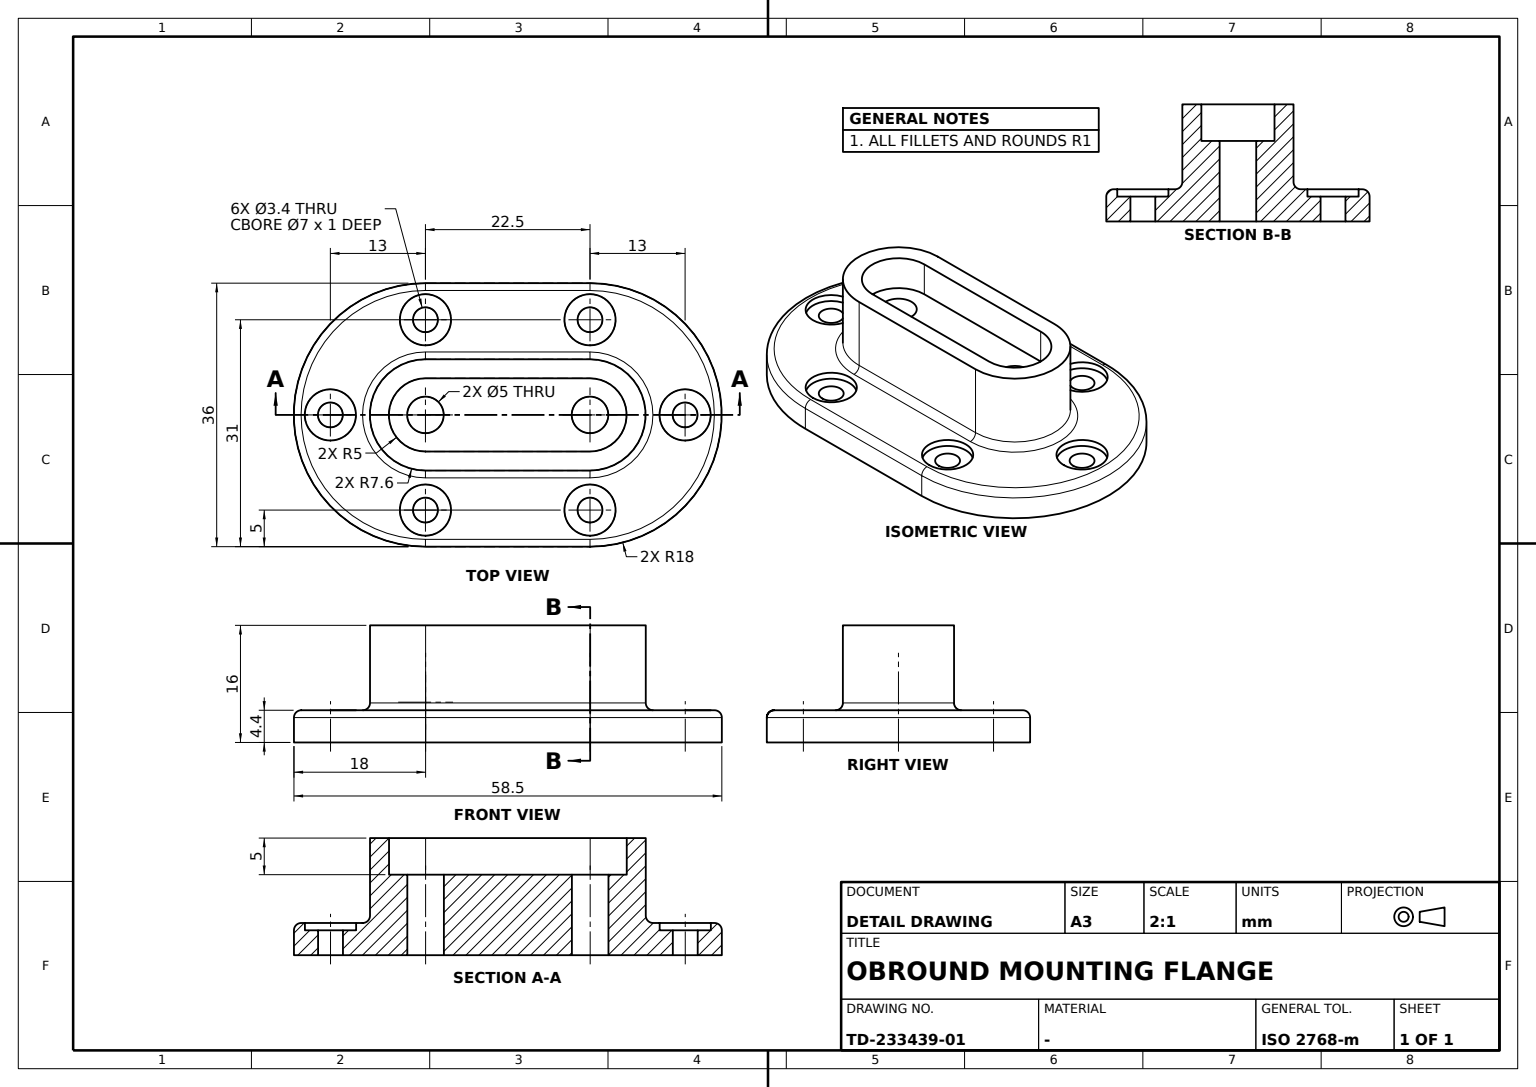
ISO-10303-21;
HEADER;
FILE_DESCRIPTION((''),'2;1');
FILE_NAME('','',(''),(''),'','','');
FILE_SCHEMA(('AUTOMOTIVE_DESIGN'));
ENDSEC;
DATA;
#1=APPLICATION_CONTEXT('');
#2=PRODUCT_CONTEXT('',#1,'mechanical');
#3=PRODUCT('','','',(#2));
#4=PRODUCT_DEFINITION_FORMATION('','',#3);
#5=PRODUCT_DEFINITION_CONTEXT('',#1,'design');
#6=PRODUCT_DEFINITION('','',#4,#5);
#7=PRODUCT_DEFINITION_SHAPE('','',#6);
#8=(LENGTH_UNIT()NAMED_UNIT(*)SI_UNIT(.MILLI.,.METRE.));
#9=(NAMED_UNIT(*)PLANE_ANGLE_UNIT()SI_UNIT($,.RADIAN.));
#10=(NAMED_UNIT(*)SI_UNIT($,.STERADIAN.)SOLID_ANGLE_UNIT());
#11=UNCERTAINTY_MEASURE_WITH_UNIT(LENGTH_MEASURE(0.005),#8,'distance_accuracy_value','');
#12=(GEOMETRIC_REPRESENTATION_CONTEXT(3)GLOBAL_UNCERTAINTY_ASSIGNED_CONTEXT((#11))GLOBAL_UNIT_ASSIGNED_CONTEXT((#8,#9,#10))REPRESENTATION_CONTEXT('',''));
#13=CARTESIAN_POINT('',(-8.6,-11.25,2.2));
#14=VERTEX_POINT('',#13);
#15=CARTESIAN_POINT('',(-7.6,-11.25,3.2));
#16=VERTEX_POINT('',#15);
#17=CARTESIAN_POINT('',(-8.6,-11.25,3.2));
#18=DIRECTION('',(0.,1.,0.));
#19=DIRECTION('',(0.,0.,1.));
#20=AXIS2_PLACEMENT_3D('',#17,#18,#19);
#21=CIRCLE('',#20,1.);
#22=EDGE_CURVE('',#14,#16,#21,.F.);
#23=ORIENTED_EDGE('',*,*,#22,.F.);
#24=CARTESIAN_POINT('',(8.6,-11.25,2.2));
#25=VERTEX_POINT('',#24);
#26=CARTESIAN_POINT('',(0.,-11.25,2.2));
#27=DIRECTION('',(1.,0.,0.));
#28=AXIS2_PLACEMENT_3D('',#26,#19,#27);
#29=CIRCLE('',#28,8.6);
#30=EDGE_CURVE('',#14,#25,#29,.T.);
#31=ORIENTED_EDGE('',*,*,#30,.T.);
#32=CARTESIAN_POINT('',(7.6,-11.25,3.2));
#33=VERTEX_POINT('',#32);
#34=CARTESIAN_POINT('',(8.6,-11.25,3.2));
#35=AXIS2_PLACEMENT_3D('',#34,#18,#19);
#36=CIRCLE('',#35,1.);
#37=EDGE_CURVE('',#25,#33,#36,.T.);
#38=ORIENTED_EDGE('',*,*,#37,.T.);
#39=CARTESIAN_POINT('',(0.,-11.25,3.2));
#40=AXIS2_PLACEMENT_3D('',#39,#19,#27);
#41=CIRCLE('',#40,7.6);
#42=EDGE_CURVE('',#16,#33,#41,.T.);
#43=ORIENTED_EDGE('',*,*,#42,.F.);
#44=EDGE_LOOP('',(#23,#31,#38,#43));
#45=FACE_BOUND('',#44,.T.);
#46=DIRECTION('',(-0.691222874,0.722641639,0.));
#47=AXIS2_PLACEMENT_3D('',#39,#19,#46);
#48=TOROIDAL_SURFACE('',#47,8.6,1.);
#49=ADVANCED_FACE('',(#45),#48,.F.);
#50=CARTESIAN_POINT('',(7.6,11.25,3.2));
#51=VERTEX_POINT('',#50);
#52=CARTESIAN_POINT('',(7.6,11.25,13.8));
#53=VERTEX_POINT('',#52);
#54=CARTESIAN_POINT('',(7.6,11.25,8.));
#55=VECTOR('',#19,1000.);
#56=LINE('',#54,#55);
#57=EDGE_CURVE('',#51,#53,#56,.T.);
#58=ORIENTED_EDGE('',*,*,#57,.T.);
#59=CARTESIAN_POINT('',(7.6,-11.25,13.8));
#60=VERTEX_POINT('',#59);
#61=CARTESIAN_POINT('',(7.6,0.,13.8));
#62=VECTOR('',#18,1000.);
#63=LINE('',#61,#62);
#64=EDGE_CURVE('',#60,#53,#63,.T.);
#65=ORIENTED_EDGE('',*,*,#64,.F.);
#66=CARTESIAN_POINT('',(7.6,-11.25,8.));
#67=LINE('',#66,#55);
#68=EDGE_CURVE('',#33,#60,#67,.T.);
#69=ORIENTED_EDGE('',*,*,#68,.F.);
#70=CARTESIAN_POINT('',(7.6,0.,3.2));
#71=LINE('',#70,#62);
#72=EDGE_CURVE('',#33,#51,#71,.T.);
#73=ORIENTED_EDGE('',*,*,#72,.T.);
#74=EDGE_LOOP('',(#58,#65,#69,#73));
#75=FACE_BOUND('',#74,.T.);
#76=CARTESIAN_POINT('',(7.6,-11.25,2.2));
#77=AXIS2_PLACEMENT_3D('',#76,#27,#18);
#78=PLANE('',#77);
#79=ADVANCED_FACE('',(#75),#78,.T.);
#80=CARTESIAN_POINT('',(2.5,-11.25,-2.2));
#81=VERTEX_POINT('',#80);
#82=CARTESIAN_POINT('',(0.,-11.25,-2.2));
#83=AXIS2_PLACEMENT_3D('',#82,#19,#27);
#84=CIRCLE('',#83,2.5);
#85=EDGE_CURVE('',#81,#81,#84,.T.);
#86=ORIENTED_EDGE('',*,*,#85,.T.);
#87=EDGE_LOOP('',(#86));
#88=FACE_BOUND('',#87,.T.);
#89=CARTESIAN_POINT('',(1.7,24.25,-2.2));
#90=VERTEX_POINT('',#89);
#91=CARTESIAN_POINT('',(0.,24.25,-2.2));
#92=AXIS2_PLACEMENT_3D('',#91,#19,#27);
#93=CIRCLE('',#92,1.7);
#94=EDGE_CURVE('',#90,#90,#93,.T.);
#95=ORIENTED_EDGE('',*,*,#94,.T.);
#96=EDGE_LOOP('',(#95));
#97=FACE_BOUND('',#96,.T.);
#98=CARTESIAN_POINT('',(2.5,11.25,-2.2));
#99=VERTEX_POINT('',#98);
#100=CARTESIAN_POINT('',(0.,11.25,-2.2));
#101=AXIS2_PLACEMENT_3D('',#100,#19,#27);
#102=CIRCLE('',#101,2.5);
#103=EDGE_CURVE('',#99,#99,#102,.T.);
#104=ORIENTED_EDGE('',*,*,#103,.T.);
#105=EDGE_LOOP('',(#104));
#106=FACE_BOUND('',#105,.T.);
#107=CARTESIAN_POINT('',(-11.3,11.25,-2.2));
#108=VERTEX_POINT('',#107);
#109=CARTESIAN_POINT('',(-13.,11.25,-2.2));
#110=AXIS2_PLACEMENT_3D('',#109,#19,#27);
#111=CIRCLE('',#110,1.7);
#112=EDGE_CURVE('',#108,#108,#111,.T.);
#113=ORIENTED_EDGE('',*,*,#112,.T.);
#114=EDGE_LOOP('',(#113));
#115=FACE_BOUND('',#114,.T.);
#116=CARTESIAN_POINT('',(14.7,11.25,-2.2));
#117=VERTEX_POINT('',#116);
#118=CARTESIAN_POINT('',(13.,11.25,-2.2));
#119=AXIS2_PLACEMENT_3D('',#118,#19,#27);
#120=CIRCLE('',#119,1.7);
#121=EDGE_CURVE('',#117,#117,#120,.T.);
#122=ORIENTED_EDGE('',*,*,#121,.T.);
#123=EDGE_LOOP('',(#122));
#124=FACE_BOUND('',#123,.T.);
#125=CARTESIAN_POINT('',(1.7,-24.25,-2.2));
#126=VERTEX_POINT('',#125);
#127=CARTESIAN_POINT('',(0.,-24.25,-2.2));
#128=AXIS2_PLACEMENT_3D('',#127,#19,#27);
#129=CIRCLE('',#128,1.7);
#130=EDGE_CURVE('',#126,#126,#129,.T.);
#131=ORIENTED_EDGE('',*,*,#130,.T.);
#132=EDGE_LOOP('',(#131));
#133=FACE_BOUND('',#132,.T.);
#134=CARTESIAN_POINT('',(14.7,-11.25,-2.2));
#135=VERTEX_POINT('',#134);
#136=CARTESIAN_POINT('',(13.,-11.25,-2.2));
#137=AXIS2_PLACEMENT_3D('',#136,#19,#27);
#138=CIRCLE('',#137,1.7);
#139=EDGE_CURVE('',#135,#135,#138,.T.);
#140=ORIENTED_EDGE('',*,*,#139,.T.);
#141=EDGE_LOOP('',(#140));
#142=FACE_BOUND('',#141,.T.);
#143=CARTESIAN_POINT('',(-11.3,-11.25,-2.2));
#144=VERTEX_POINT('',#143);
#145=CARTESIAN_POINT('',(-13.,-11.25,-2.2));
#146=AXIS2_PLACEMENT_3D('',#145,#19,#27);
#147=CIRCLE('',#146,1.7);
#148=EDGE_CURVE('',#144,#144,#147,.T.);
#149=ORIENTED_EDGE('',*,*,#148,.T.);
#150=EDGE_LOOP('',(#149));
#151=FACE_BOUND('',#150,.T.);
#152=CARTESIAN_POINT('',(-18.,-11.25,-2.2));
#153=VERTEX_POINT('',#152);
#154=CARTESIAN_POINT('',(18.,-11.25,-2.2));
#155=VERTEX_POINT('',#154);
#156=CIRCLE('',#83,18.);
#157=EDGE_CURVE('',#153,#155,#156,.T.);
#158=ORIENTED_EDGE('',*,*,#157,.F.);
#159=CARTESIAN_POINT('',(-18.,11.25,-2.2));
#160=VERTEX_POINT('',#159);
#161=CARTESIAN_POINT('',(-18.,0.,-2.2));
#162=LINE('',#161,#62);
#163=EDGE_CURVE('',#153,#160,#162,.T.);
#164=ORIENTED_EDGE('',*,*,#163,.T.);
#165=CARTESIAN_POINT('',(18.,11.25,-2.2));
#166=VERTEX_POINT('',#165);
#167=CIRCLE('',#101,18.);
#168=EDGE_CURVE('',#166,#160,#167,.T.);
#169=ORIENTED_EDGE('',*,*,#168,.F.);
#170=CARTESIAN_POINT('',(18.,0.,-2.2));
#171=LINE('',#170,#62);
#172=EDGE_CURVE('',#155,#166,#171,.T.);
#173=ORIENTED_EDGE('',*,*,#172,.F.);
#174=EDGE_LOOP('',(#158,#164,#169,#173));
#175=FACE_BOUND('',#174,.T.);
#176=CARTESIAN_POINT('',(0.,0.,-2.2));
#177=AXIS2_PLACEMENT_3D('',#176,#19,#18);
#178=PLANE('',#177);
#179=ADVANCED_FACE('',(#88,#97,#106,#115,#124,#133,#142,#151,#175),#178,.F.);
#180=CARTESIAN_POINT('',(3.5,-24.25,1.2));
#181=VERTEX_POINT('',#180);
#182=CARTESIAN_POINT('',(0.,-24.25,1.2));
#183=AXIS2_PLACEMENT_3D('',#182,#19,#27);
#184=CIRCLE('',#183,3.5);
#185=EDGE_CURVE('',#181,#181,#184,.T.);
#186=ORIENTED_EDGE('',*,*,#185,.F.);
#187=EDGE_LOOP('',(#186));
#188=FACE_BOUND('',#187,.T.);
#189=CARTESIAN_POINT('',(3.5,-24.25,2.2));
#190=VERTEX_POINT('',#189);
#191=CARTESIAN_POINT('',(0.,-24.25,2.2));
#192=AXIS2_PLACEMENT_3D('',#191,#19,#27);
#193=CIRCLE('',#192,3.5);
#194=EDGE_CURVE('',#190,#190,#193,.T.);
#195=ORIENTED_EDGE('',*,*,#194,.T.);
#196=EDGE_LOOP('',(#195));
#197=FACE_BOUND('',#196,.T.);
#198=CARTESIAN_POINT('',(0.,-24.25,1.7));
#199=AXIS2_PLACEMENT_3D('',#198,#19,#18);
#200=CYLINDRICAL_SURFACE('',#199,3.5);
#201=ADVANCED_FACE('',(#188,#197),#200,.F.);
#202=CARTESIAN_POINT('',(-18.,-11.25,1.2));
#203=VERTEX_POINT('',#202);
#204=CARTESIAN_POINT('',(-18.,11.25,1.2));
#205=VERTEX_POINT('',#204);
#206=CARTESIAN_POINT('',(-18.,0.,1.2));
#207=LINE('',#206,#62);
#208=EDGE_CURVE('',#203,#205,#207,.T.);
#209=ORIENTED_EDGE('',*,*,#208,.T.);
#210=CARTESIAN_POINT('',(-18.,11.25,0.));
#211=LINE('',#210,#55);
#212=EDGE_CURVE('',#160,#205,#211,.T.);
#213=ORIENTED_EDGE('',*,*,#212,.F.);
#214=ORIENTED_EDGE('',*,*,#163,.F.);
#215=CARTESIAN_POINT('',(-18.,-11.25,0.));
#216=LINE('',#215,#55);
#217=EDGE_CURVE('',#153,#203,#216,.T.);
#218=ORIENTED_EDGE('',*,*,#217,.T.);
#219=EDGE_LOOP('',(#209,#213,#214,#218));
#220=FACE_BOUND('',#219,.T.);
#221=AXIS2_PLACEMENT_3D('',#215,#27,#18);
#222=PLANE('',#221);
#223=ADVANCED_FACE('',(#220),#222,.F.);
#224=CARTESIAN_POINT('',(16.5,11.25,1.2));
#225=VERTEX_POINT('',#224);
#226=CARTESIAN_POINT('',(13.,11.25,1.2));
#227=AXIS2_PLACEMENT_3D('',#226,#19,#27);
#228=CIRCLE('',#227,3.5);
#229=EDGE_CURVE('',#225,#225,#228,.T.);
#230=ORIENTED_EDGE('',*,*,#229,.F.);
#231=EDGE_LOOP('',(#230));
#232=FACE_BOUND('',#231,.T.);
#233=CARTESIAN_POINT('',(16.5,11.25,2.2));
#234=VERTEX_POINT('',#233);
#235=CARTESIAN_POINT('',(13.,11.25,2.2));
#236=AXIS2_PLACEMENT_3D('',#235,#19,#27);
#237=CIRCLE('',#236,3.5);
#238=EDGE_CURVE('',#234,#234,#237,.T.);
#239=ORIENTED_EDGE('',*,*,#238,.T.);
#240=EDGE_LOOP('',(#239));
#241=FACE_BOUND('',#240,.T.);
#242=CARTESIAN_POINT('',(13.,11.25,1.7));
#243=AXIS2_PLACEMENT_3D('',#242,#19,#18);
#244=CYLINDRICAL_SURFACE('',#243,3.5);
#245=ADVANCED_FACE('',(#232,#241),#244,.F.);
#246=ORIENTED_EDGE('',*,*,#212,.T.);
#247=CARTESIAN_POINT('',(18.,11.25,1.2));
#248=VERTEX_POINT('',#247);
#249=CARTESIAN_POINT('',(0.,11.25,1.2));
#250=AXIS2_PLACEMENT_3D('',#249,#19,#27);
#251=CIRCLE('',#250,18.);
#252=EDGE_CURVE('',#248,#205,#251,.T.);
#253=ORIENTED_EDGE('',*,*,#252,.F.);
#254=CARTESIAN_POINT('',(18.,11.25,0.));
#255=LINE('',#254,#55);
#256=EDGE_CURVE('',#166,#248,#255,.T.);
#257=ORIENTED_EDGE('',*,*,#256,.F.);
#258=ORIENTED_EDGE('',*,*,#168,.T.);
#259=EDGE_LOOP('',(#246,#253,#257,#258));
#260=FACE_BOUND('',#259,.T.);
#261=CARTESIAN_POINT('',(0.,11.25,0.));
#262=AXIS2_PLACEMENT_3D('',#261,#19,#18);
#263=CYLINDRICAL_SURFACE('',#262,18.);
#264=ADVANCED_FACE('',(#260),#263,.T.);
#265=CARTESIAN_POINT('',(-11.3,11.25,1.2));
#266=VERTEX_POINT('',#265);
#267=CARTESIAN_POINT('',(-13.,11.25,1.2));
#268=AXIS2_PLACEMENT_3D('',#267,#19,#27);
#269=CIRCLE('',#268,1.7);
#270=EDGE_CURVE('',#266,#266,#269,.T.);
#271=ORIENTED_EDGE('',*,*,#270,.T.);
#272=EDGE_LOOP('',(#271));
#273=FACE_BOUND('',#272,.T.);
#274=ORIENTED_EDGE('',*,*,#112,.F.);
#275=EDGE_LOOP('',(#274));
#276=FACE_BOUND('',#275,.T.);
#277=CARTESIAN_POINT('',(-13.,11.25,-1.16));
#278=AXIS2_PLACEMENT_3D('',#277,#19,#18);
#279=CYLINDRICAL_SURFACE('',#278,1.7);
#280=ADVANCED_FACE('',(#273,#276),#279,.F.);
#281=ORIENTED_EDGE('',*,*,#72,.F.);
#282=ORIENTED_EDGE('',*,*,#37,.F.);
#283=CARTESIAN_POINT('',(8.6,11.25,2.2));
#284=VERTEX_POINT('',#283);
#285=CARTESIAN_POINT('',(8.6,0.,2.2));
#286=LINE('',#285,#62);
#287=EDGE_CURVE('',#25,#284,#286,.T.);
#288=ORIENTED_EDGE('',*,*,#287,.T.);
#289=CARTESIAN_POINT('',(8.6,11.25,3.2));
#290=AXIS2_PLACEMENT_3D('',#289,#18,#19);
#291=CIRCLE('',#290,1.);
#292=EDGE_CURVE('',#284,#51,#291,.T.);
#293=ORIENTED_EDGE('',*,*,#292,.T.);
#294=EDGE_LOOP('',(#281,#282,#288,#293));
#295=FACE_BOUND('',#294,.T.);
#296=CARTESIAN_POINT('',(8.6,0.,3.2));
#297=DIRECTION('',(0.,0.,-1.));
#298=AXIS2_PLACEMENT_3D('',#296,#18,#297);
#299=CYLINDRICAL_SURFACE('',#298,1.);
#300=ADVANCED_FACE('',(#295),#299,.F.);
#301=CARTESIAN_POINT('',(17.,11.25,2.2));
#302=VERTEX_POINT('',#301);
#303=CARTESIAN_POINT('',(-17.,11.25,2.2));
#304=VERTEX_POINT('',#303);
#305=CARTESIAN_POINT('',(0.,11.25,2.2));
#306=AXIS2_PLACEMENT_3D('',#305,#19,#27);
#307=CIRCLE('',#306,17.);
#308=EDGE_CURVE('',#302,#304,#307,.T.);
#309=ORIENTED_EDGE('',*,*,#308,.F.);
#310=CARTESIAN_POINT('',(17.,11.25,1.2));
#311=DIRECTION('',(0.,-1.,0.));
#312=AXIS2_PLACEMENT_3D('',#310,#311,#297);
#313=CIRCLE('',#312,1.);
#314=EDGE_CURVE('',#248,#302,#313,.T.);
#315=ORIENTED_EDGE('',*,*,#314,.F.);
#316=ORIENTED_EDGE('',*,*,#252,.T.);
#317=CARTESIAN_POINT('',(-17.,11.25,1.2));
#318=AXIS2_PLACEMENT_3D('',#317,#18,#19);
#319=CIRCLE('',#318,1.);
#320=EDGE_CURVE('',#205,#304,#319,.T.);
#321=ORIENTED_EDGE('',*,*,#320,.T.);
#322=EDGE_LOOP('',(#309,#315,#316,#321));
#323=FACE_BOUND('',#322,.T.);
#324=DIRECTION('',(0.579361636,-0.815070608,0.));
#325=AXIS2_PLACEMENT_3D('',#249,#19,#324);
#326=TOROIDAL_SURFACE('',#325,17.,1.);
#327=ADVANCED_FACE('',(#323),#326,.T.);
#328=ORIENTED_EDGE('',*,*,#229,.T.);
#329=EDGE_LOOP('',(#328));
#330=FACE_BOUND('',#329,.T.);
#331=CARTESIAN_POINT('',(14.7,11.25,1.2));
#332=VERTEX_POINT('',#331);
#333=CIRCLE('',#227,1.7);
#334=EDGE_CURVE('',#332,#332,#333,.T.);
#335=ORIENTED_EDGE('',*,*,#334,.F.);
#336=EDGE_LOOP('',(#335));
#337=FACE_BOUND('',#336,.T.);
#338=CARTESIAN_POINT('',(0.,0.,1.2));
#339=AXIS2_PLACEMENT_3D('',#338,#19,#18);
#340=PLANE('',#339);
#341=ADVANCED_FACE('',(#330,#337),#340,.T.);
#342=CARTESIAN_POINT('',(1.7,-24.25,1.2));
#343=VERTEX_POINT('',#342);
#344=CIRCLE('',#183,1.7);
#345=EDGE_CURVE('',#343,#343,#344,.T.);
#346=ORIENTED_EDGE('',*,*,#345,.F.);
#347=EDGE_LOOP('',(#346));
#348=FACE_BOUND('',#347,.T.);
#349=ORIENTED_EDGE('',*,*,#185,.T.);
#350=EDGE_LOOP('',(#349));
#351=FACE_BOUND('',#350,.T.);
#352=ADVANCED_FACE('',(#348,#351),#340,.T.);
#353=CARTESIAN_POINT('',(-7.6,11.25,3.2));
#354=VERTEX_POINT('',#353);
#355=CARTESIAN_POINT('',(0.,11.25,3.2));
#356=AXIS2_PLACEMENT_3D('',#355,#19,#27);
#357=CIRCLE('',#356,7.6);
#358=EDGE_CURVE('',#51,#354,#357,.T.);
#359=ORIENTED_EDGE('',*,*,#358,.F.);
#360=ORIENTED_EDGE('',*,*,#292,.F.);
#361=CARTESIAN_POINT('',(-8.6,11.25,2.2));
#362=VERTEX_POINT('',#361);
#363=CIRCLE('',#306,8.6);
#364=EDGE_CURVE('',#284,#362,#363,.T.);
#365=ORIENTED_EDGE('',*,*,#364,.T.);
#366=CARTESIAN_POINT('',(-8.6,11.25,3.2));
#367=AXIS2_PLACEMENT_3D('',#366,#18,#19);
#368=CIRCLE('',#367,1.);
#369=EDGE_CURVE('',#362,#354,#368,.F.);
#370=ORIENTED_EDGE('',*,*,#369,.T.);
#371=EDGE_LOOP('',(#359,#360,#365,#370));
#372=FACE_BOUND('',#371,.T.);
#373=DIRECTION('',(0.514465485,-0.857511088,0.));
#374=AXIS2_PLACEMENT_3D('',#355,#19,#373);
#375=TOROIDAL_SURFACE('',#374,8.6,1.);
#376=ADVANCED_FACE('',(#372),#375,.F.);
#377=ORIENTED_EDGE('',*,*,#334,.T.);
#378=EDGE_LOOP('',(#377));
#379=FACE_BOUND('',#378,.T.);
#380=ORIENTED_EDGE('',*,*,#121,.F.);
#381=EDGE_LOOP('',(#380));
#382=FACE_BOUND('',#381,.T.);
#383=CARTESIAN_POINT('',(13.,11.25,-1.16));
#384=AXIS2_PLACEMENT_3D('',#383,#19,#18);
#385=CYLINDRICAL_SURFACE('',#384,1.7);
#386=ADVANCED_FACE('',(#379,#382),#385,.F.);
#387=CARTESIAN_POINT('',(16.5,-11.25,1.2));
#388=VERTEX_POINT('',#387);
#389=CARTESIAN_POINT('',(13.,-11.25,1.2));
#390=AXIS2_PLACEMENT_3D('',#389,#19,#27);
#391=CIRCLE('',#390,3.5);
#392=EDGE_CURVE('',#388,#388,#391,.T.);
#393=ORIENTED_EDGE('',*,*,#392,.T.);
#394=EDGE_LOOP('',(#393));
#395=FACE_BOUND('',#394,.T.);
#396=CARTESIAN_POINT('',(14.7,-11.25,1.2));
#397=VERTEX_POINT('',#396);
#398=CIRCLE('',#390,1.7);
#399=EDGE_CURVE('',#397,#397,#398,.T.);
#400=ORIENTED_EDGE('',*,*,#399,.F.);
#401=EDGE_LOOP('',(#400));
#402=FACE_BOUND('',#401,.T.);
#403=ADVANCED_FACE('',(#395,#402),#340,.T.);
#404=CARTESIAN_POINT('',(5.,11.25,8.8));
#405=VERTEX_POINT('',#404);
#406=CARTESIAN_POINT('',(5.,11.25,13.8));
#407=VERTEX_POINT('',#406);
#408=CARTESIAN_POINT('',(5.,11.25,8.));
#409=LINE('',#408,#55);
#410=EDGE_CURVE('',#405,#407,#409,.T.);
#411=ORIENTED_EDGE('',*,*,#410,.F.);
#412=CARTESIAN_POINT('',(5.,-11.25,8.8));
#413=VERTEX_POINT('',#412);
#414=CARTESIAN_POINT('',(5.,0.,8.8));
#415=LINE('',#414,#62);
#416=EDGE_CURVE('',#413,#405,#415,.T.);
#417=ORIENTED_EDGE('',*,*,#416,.F.);
#418=CARTESIAN_POINT('',(5.,-11.25,13.8));
#419=VERTEX_POINT('',#418);
#420=CARTESIAN_POINT('',(5.,-11.25,8.));
#421=LINE('',#420,#55);
#422=EDGE_CURVE('',#413,#419,#421,.T.);
#423=ORIENTED_EDGE('',*,*,#422,.T.);
#424=CARTESIAN_POINT('',(5.,0.,13.8));
#425=LINE('',#424,#62);
#426=EDGE_CURVE('',#419,#407,#425,.T.);
#427=ORIENTED_EDGE('',*,*,#426,.T.);
#428=EDGE_LOOP('',(#411,#417,#423,#427));
#429=FACE_BOUND('',#428,.T.);
#430=CARTESIAN_POINT('',(5.,-11.25,2.2));
#431=AXIS2_PLACEMENT_3D('',#430,#27,#18);
#432=PLANE('',#431);
#433=ADVANCED_FACE('',(#429),#432,.F.);
#434=CARTESIAN_POINT('',(-17.,-11.25,2.2));
#435=VERTEX_POINT('',#434);
#436=CARTESIAN_POINT('',(-17.,-11.25,1.2));
#437=AXIS2_PLACEMENT_3D('',#436,#18,#19);
#438=CIRCLE('',#437,1.);
#439=EDGE_CURVE('',#203,#435,#438,.T.);
#440=ORIENTED_EDGE('',*,*,#439,.T.);
#441=CARTESIAN_POINT('',(-17.,0.,2.2));
#442=LINE('',#441,#62);
#443=EDGE_CURVE('',#435,#304,#442,.T.);
#444=ORIENTED_EDGE('',*,*,#443,.T.);
#445=ORIENTED_EDGE('',*,*,#320,.F.);
#446=ORIENTED_EDGE('',*,*,#208,.F.);
#447=EDGE_LOOP('',(#440,#444,#445,#446));
#448=FACE_BOUND('',#447,.T.);
#449=CARTESIAN_POINT('',(-17.,0.,1.2));
#450=DIRECTION('',(-1.,0.,0.));
#451=AXIS2_PLACEMENT_3D('',#449,#18,#450);
#452=CYLINDRICAL_SURFACE('',#451,1.);
#453=ADVANCED_FACE('',(#448),#452,.T.);
#454=CARTESIAN_POINT('',(-7.6,-11.25,13.8));
#455=VERTEX_POINT('',#454);
#456=CARTESIAN_POINT('',(-7.6,11.25,13.8));
#457=VERTEX_POINT('',#456);
#458=CARTESIAN_POINT('',(-7.6,0.,13.8));
#459=LINE('',#458,#62);
#460=EDGE_CURVE('',#455,#457,#459,.T.);
#461=ORIENTED_EDGE('',*,*,#460,.T.);
#462=CARTESIAN_POINT('',(-7.6,11.25,8.));
#463=LINE('',#462,#55);
#464=EDGE_CURVE('',#354,#457,#463,.T.);
#465=ORIENTED_EDGE('',*,*,#464,.F.);
#466=CARTESIAN_POINT('',(-7.6,0.,3.2));
#467=LINE('',#466,#62);
#468=EDGE_CURVE('',#16,#354,#467,.T.);
#469=ORIENTED_EDGE('',*,*,#468,.F.);
#470=CARTESIAN_POINT('',(-7.6,-11.25,8.));
#471=LINE('',#470,#55);
#472=EDGE_CURVE('',#16,#455,#471,.T.);
#473=ORIENTED_EDGE('',*,*,#472,.T.);
#474=EDGE_LOOP('',(#461,#465,#469,#473));
#475=FACE_BOUND('',#474,.T.);
#476=CARTESIAN_POINT('',(-7.6,-11.25,2.2));
#477=AXIS2_PLACEMENT_3D('',#476,#27,#18);
#478=PLANE('',#477);
#479=ADVANCED_FACE('',(#475),#478,.F.);
#480=CARTESIAN_POINT('',(-9.5,-11.25,1.2));
#481=VERTEX_POINT('',#480);
#482=CARTESIAN_POINT('',(-13.,-11.25,1.2));
#483=AXIS2_PLACEMENT_3D('',#482,#19,#27);
#484=CIRCLE('',#483,3.5);
#485=EDGE_CURVE('',#481,#481,#484,.T.);
#486=ORIENTED_EDGE('',*,*,#485,.F.);
#487=EDGE_LOOP('',(#486));
#488=FACE_BOUND('',#487,.T.);
#489=CARTESIAN_POINT('',(-9.5,-11.25,2.2));
#490=VERTEX_POINT('',#489);
#491=CARTESIAN_POINT('',(-13.,-11.25,2.2));
#492=AXIS2_PLACEMENT_3D('',#491,#19,#27);
#493=CIRCLE('',#492,3.5);
#494=EDGE_CURVE('',#490,#490,#493,.T.);
#495=ORIENTED_EDGE('',*,*,#494,.T.);
#496=EDGE_LOOP('',(#495));
#497=FACE_BOUND('',#496,.T.);
#498=CARTESIAN_POINT('',(-13.,-11.25,1.7));
#499=AXIS2_PLACEMENT_3D('',#498,#19,#18);
#500=CYLINDRICAL_SURFACE('',#499,3.5);
#501=ADVANCED_FACE('',(#488,#497),#500,.F.);
#502=ORIENTED_EDGE('',*,*,#57,.F.);
#503=ORIENTED_EDGE('',*,*,#358,.T.);
#504=ORIENTED_EDGE('',*,*,#464,.T.);
#505=CARTESIAN_POINT('',(0.,11.25,13.8));
#506=AXIS2_PLACEMENT_3D('',#505,#19,#27);
#507=CIRCLE('',#506,7.6);
#508=EDGE_CURVE('',#53,#457,#507,.T.);
#509=ORIENTED_EDGE('',*,*,#508,.F.);
#510=EDGE_LOOP('',(#502,#503,#504,#509));
#511=FACE_BOUND('',#510,.T.);
#512=CARTESIAN_POINT('',(0.,11.25,8.));
#513=AXIS2_PLACEMENT_3D('',#512,#19,#18);
#514=CYLINDRICAL_SURFACE('',#513,7.6);
#515=ADVANCED_FACE('',(#511),#514,.T.);
#516=ORIENTED_EDGE('',*,*,#345,.T.);
#517=EDGE_LOOP('',(#516));
#518=FACE_BOUND('',#517,.T.);
#519=ORIENTED_EDGE('',*,*,#130,.F.);
#520=EDGE_LOOP('',(#519));
#521=FACE_BOUND('',#520,.T.);
#522=CARTESIAN_POINT('',(0.,-24.25,-1.16));
#523=AXIS2_PLACEMENT_3D('',#522,#19,#18);
#524=CYLINDRICAL_SURFACE('',#523,1.7);
#525=ADVANCED_FACE('',(#518,#521),#524,.F.);
#526=ORIENTED_EDGE('',*,*,#314,.T.);
#527=CARTESIAN_POINT('',(17.,-11.25,2.2));
#528=VERTEX_POINT('',#527);
#529=CARTESIAN_POINT('',(17.,0.,2.2));
#530=VECTOR('',#311,1000.);
#531=LINE('',#529,#530);
#532=EDGE_CURVE('',#302,#528,#531,.T.);
#533=ORIENTED_EDGE('',*,*,#532,.T.);
#534=CARTESIAN_POINT('',(18.,-11.25,1.2));
#535=VERTEX_POINT('',#534);
#536=CARTESIAN_POINT('',(17.,-11.25,1.2));
#537=AXIS2_PLACEMENT_3D('',#536,#311,#297);
#538=CIRCLE('',#537,1.);
#539=EDGE_CURVE('',#535,#528,#538,.T.);
#540=ORIENTED_EDGE('',*,*,#539,.F.);
#541=CARTESIAN_POINT('',(18.,0.,1.2));
#542=LINE('',#541,#530);
#543=EDGE_CURVE('',#248,#535,#542,.T.);
#544=ORIENTED_EDGE('',*,*,#543,.F.);
#545=EDGE_LOOP('',(#526,#533,#540,#544));
#546=FACE_BOUND('',#545,.T.);
#547=CARTESIAN_POINT('',(17.,0.,1.2));
#548=AXIS2_PLACEMENT_3D('',#547,#311,#27);
#549=CYLINDRICAL_SURFACE('',#548,1.);
#550=ADVANCED_FACE('',(#546),#549,.T.);
#551=CARTESIAN_POINT('',(1.7,24.25,1.2));
#552=VERTEX_POINT('',#551);
#553=CARTESIAN_POINT('',(0.,24.25,1.2));
#554=AXIS2_PLACEMENT_3D('',#553,#19,#27);
#555=CIRCLE('',#554,1.7);
#556=EDGE_CURVE('',#552,#552,#555,.T.);
#557=ORIENTED_EDGE('',*,*,#556,.T.);
#558=EDGE_LOOP('',(#557));
#559=FACE_BOUND('',#558,.T.);
#560=ORIENTED_EDGE('',*,*,#94,.F.);
#561=EDGE_LOOP('',(#560));
#562=FACE_BOUND('',#561,.T.);
#563=CARTESIAN_POINT('',(0.,24.25,-1.16));
#564=AXIS2_PLACEMENT_3D('',#563,#19,#18);
#565=CYLINDRICAL_SURFACE('',#564,1.7);
#566=ADVANCED_FACE('',(#559,#562),#565,.F.);
#567=ORIENTED_EDGE('',*,*,#399,.T.);
#568=EDGE_LOOP('',(#567));
#569=FACE_BOUND('',#568,.T.);
#570=ORIENTED_EDGE('',*,*,#139,.F.);
#571=EDGE_LOOP('',(#570));
#572=FACE_BOUND('',#571,.T.);
#573=CARTESIAN_POINT('',(13.,-11.25,-1.16));
#574=AXIS2_PLACEMENT_3D('',#573,#19,#18);
#575=CYLINDRICAL_SURFACE('',#574,1.7);
#576=ADVANCED_FACE('',(#569,#572),#575,.F.);
#577=CARTESIAN_POINT('',(-5.,-11.25,8.8));
#578=VERTEX_POINT('',#577);
#579=CARTESIAN_POINT('',(0.,-11.25,8.8));
#580=AXIS2_PLACEMENT_3D('',#579,#19,#27);
#581=CIRCLE('',#580,5.);
#582=EDGE_CURVE('',#578,#413,#581,.T.);
#583=ORIENTED_EDGE('',*,*,#582,.F.);
#584=CARTESIAN_POINT('',(-5.,-11.25,13.8));
#585=VERTEX_POINT('',#584);
#586=CARTESIAN_POINT('',(-5.,-11.25,8.));
#587=LINE('',#586,#55);
#588=EDGE_CURVE('',#578,#585,#587,.T.);
#589=ORIENTED_EDGE('',*,*,#588,.T.);
#590=CARTESIAN_POINT('',(0.,-11.25,13.8));
#591=AXIS2_PLACEMENT_3D('',#590,#19,#27);
#592=CIRCLE('',#591,5.);
#593=EDGE_CURVE('',#585,#419,#592,.T.);
#594=ORIENTED_EDGE('',*,*,#593,.T.);
#595=ORIENTED_EDGE('',*,*,#422,.F.);
#596=EDGE_LOOP('',(#583,#589,#594,#595));
#597=FACE_BOUND('',#596,.T.);
#598=CARTESIAN_POINT('',(0.,-11.25,8.));
#599=AXIS2_PLACEMENT_3D('',#598,#19,#18);
#600=CYLINDRICAL_SURFACE('',#599,5.);
#601=ADVANCED_FACE('',(#597),#600,.F.);
#602=ORIENTED_EDGE('',*,*,#426,.F.);
#603=ORIENTED_EDGE('',*,*,#593,.F.);
#604=CARTESIAN_POINT('',(-5.,11.25,13.8));
#605=VERTEX_POINT('',#604);
#606=CARTESIAN_POINT('',(-5.,0.,13.8));
#607=LINE('',#606,#62);
#608=EDGE_CURVE('',#585,#605,#607,.T.);
#609=ORIENTED_EDGE('',*,*,#608,.T.);
#610=CIRCLE('',#506,5.);
#611=EDGE_CURVE('',#407,#605,#610,.T.);
#612=ORIENTED_EDGE('',*,*,#611,.F.);
#613=EDGE_LOOP('',(#602,#603,#609,#612));
#614=FACE_BOUND('',#613,.T.);
#615=ORIENTED_EDGE('',*,*,#508,.T.);
#616=ORIENTED_EDGE('',*,*,#460,.F.);
#617=CIRCLE('',#591,7.6);
#618=EDGE_CURVE('',#455,#60,#617,.T.);
#619=ORIENTED_EDGE('',*,*,#618,.T.);
#620=ORIENTED_EDGE('',*,*,#64,.T.);
#621=EDGE_LOOP('',(#615,#616,#619,#620));
#622=FACE_BOUND('',#621,.T.);
#623=CARTESIAN_POINT('',(0.,0.,13.8));
#624=AXIS2_PLACEMENT_3D('',#623,#19,#18);
#625=PLANE('',#624);
#626=ADVANCED_FACE('',(#614,#622),#625,.T.);
#627=ORIENTED_EDGE('',*,*,#22,.T.);
#628=ORIENTED_EDGE('',*,*,#468,.T.);
#629=ORIENTED_EDGE('',*,*,#369,.F.);
#630=CARTESIAN_POINT('',(-8.6,0.,2.2));
#631=LINE('',#630,#62);
#632=EDGE_CURVE('',#14,#362,#631,.T.);
#633=ORIENTED_EDGE('',*,*,#632,.F.);
#634=EDGE_LOOP('',(#627,#628,#629,#633));
#635=FACE_BOUND('',#634,.T.);
#636=CARTESIAN_POINT('',(-8.6,0.,3.2));
#637=AXIS2_PLACEMENT_3D('',#636,#18,#297);
#638=CYLINDRICAL_SURFACE('',#637,1.);
#639=ADVANCED_FACE('',(#635),#638,.F.);
#640=CARTESIAN_POINT('',(3.5,24.25,2.2));
#641=VERTEX_POINT('',#640);
#642=CARTESIAN_POINT('',(0.,24.25,2.2));
#643=AXIS2_PLACEMENT_3D('',#642,#19,#27);
#644=CIRCLE('',#643,3.5);
#645=EDGE_CURVE('',#641,#641,#644,.T.);
#646=ORIENTED_EDGE('',*,*,#645,.T.);
#647=EDGE_LOOP('',(#646));
#648=FACE_BOUND('',#647,.T.);
#649=CARTESIAN_POINT('',(3.5,24.25,1.2));
#650=VERTEX_POINT('',#649);
#651=CIRCLE('',#554,3.5);
#652=EDGE_CURVE('',#650,#650,#651,.T.);
#653=ORIENTED_EDGE('',*,*,#652,.F.);
#654=EDGE_LOOP('',(#653));
#655=FACE_BOUND('',#654,.T.);
#656=CARTESIAN_POINT('',(0.,24.25,1.7));
#657=AXIS2_PLACEMENT_3D('',#656,#19,#18);
#658=CYLINDRICAL_SURFACE('',#657,3.5);
#659=ADVANCED_FACE('',(#648,#655),#658,.F.);
#660=CARTESIAN_POINT('',(16.5,-11.25,2.2));
#661=VERTEX_POINT('',#660);
#662=CARTESIAN_POINT('',(13.,-11.25,2.2));
#663=AXIS2_PLACEMENT_3D('',#662,#19,#27);
#664=CIRCLE('',#663,3.5);
#665=EDGE_CURVE('',#661,#661,#664,.T.);
#666=ORIENTED_EDGE('',*,*,#665,.T.);
#667=EDGE_LOOP('',(#666));
#668=FACE_BOUND('',#667,.T.);
#669=ORIENTED_EDGE('',*,*,#392,.F.);
#670=EDGE_LOOP('',(#669));
#671=FACE_BOUND('',#670,.T.);
#672=CARTESIAN_POINT('',(13.,-11.25,1.7));
#673=AXIS2_PLACEMENT_3D('',#672,#19,#18);
#674=CYLINDRICAL_SURFACE('',#673,3.5);
#675=ADVANCED_FACE('',(#668,#671),#674,.F.);
#676=CARTESIAN_POINT('',(2.5,-11.25,8.8));
#677=VERTEX_POINT('',#676);
#678=CIRCLE('',#580,2.5);
#679=EDGE_CURVE('',#677,#677,#678,.T.);
#680=ORIENTED_EDGE('',*,*,#679,.F.);
#681=EDGE_LOOP('',(#680));
#682=FACE_BOUND('',#681,.T.);
#683=CARTESIAN_POINT('',(-5.,11.25,8.8));
#684=VERTEX_POINT('',#683);
#685=CARTESIAN_POINT('',(-5.,0.,8.8));
#686=LINE('',#685,#62);
#687=EDGE_CURVE('',#578,#684,#686,.T.);
#688=ORIENTED_EDGE('',*,*,#687,.F.);
#689=ORIENTED_EDGE('',*,*,#582,.T.);
#690=ORIENTED_EDGE('',*,*,#416,.T.);
#691=CARTESIAN_POINT('',(0.,11.25,8.8));
#692=AXIS2_PLACEMENT_3D('',#691,#19,#27);
#693=CIRCLE('',#692,5.);
#694=EDGE_CURVE('',#405,#684,#693,.T.);
#695=ORIENTED_EDGE('',*,*,#694,.T.);
#696=EDGE_LOOP('',(#688,#689,#690,#695));
#697=FACE_BOUND('',#696,.T.);
#698=CARTESIAN_POINT('',(2.5,11.25,8.8));
#699=VERTEX_POINT('',#698);
#700=CIRCLE('',#692,2.5);
#701=EDGE_CURVE('',#699,#699,#700,.T.);
#702=ORIENTED_EDGE('',*,*,#701,.F.);
#703=EDGE_LOOP('',(#702));
#704=FACE_BOUND('',#703,.T.);
#705=CARTESIAN_POINT('',(0.,0.,8.8));
#706=AXIS2_PLACEMENT_3D('',#705,#19,#18);
#707=PLANE('',#706);
#708=ADVANCED_FACE('',(#682,#697,#704),#707,.T.);
#709=ORIENTED_EDGE('',*,*,#238,.F.);
#710=EDGE_LOOP('',(#709));
#711=FACE_BOUND('',#710,.T.);
#712=CARTESIAN_POINT('',(-9.5,11.25,2.2));
#713=VERTEX_POINT('',#712);
#714=CARTESIAN_POINT('',(-13.,11.25,2.2));
#715=AXIS2_PLACEMENT_3D('',#714,#19,#27);
#716=CIRCLE('',#715,3.5);
#717=EDGE_CURVE('',#713,#713,#716,.T.);
#718=ORIENTED_EDGE('',*,*,#717,.F.);
#719=EDGE_LOOP('',(#718));
#720=FACE_BOUND('',#719,.T.);
#721=ORIENTED_EDGE('',*,*,#645,.F.);
#722=EDGE_LOOP('',(#721));
#723=FACE_BOUND('',#722,.T.);
#724=ORIENTED_EDGE('',*,*,#494,.F.);
#725=EDGE_LOOP('',(#724));
#726=FACE_BOUND('',#725,.T.);
#727=ORIENTED_EDGE('',*,*,#287,.F.);
#728=ORIENTED_EDGE('',*,*,#30,.F.);
#729=ORIENTED_EDGE('',*,*,#632,.T.);
#730=ORIENTED_EDGE('',*,*,#364,.F.);
#731=EDGE_LOOP('',(#727,#728,#729,#730));
#732=FACE_BOUND('',#731,.T.);
#733=ORIENTED_EDGE('',*,*,#194,.F.);
#734=EDGE_LOOP('',(#733));
#735=FACE_BOUND('',#734,.T.);
#736=ORIENTED_EDGE('',*,*,#665,.F.);
#737=EDGE_LOOP('',(#736));
#738=FACE_BOUND('',#737,.T.);
#739=ORIENTED_EDGE('',*,*,#532,.F.);
#740=ORIENTED_EDGE('',*,*,#308,.T.);
#741=ORIENTED_EDGE('',*,*,#443,.F.);
#742=CIRCLE('',#28,17.);
#743=EDGE_CURVE('',#435,#528,#742,.T.);
#744=ORIENTED_EDGE('',*,*,#743,.T.);
#745=EDGE_LOOP('',(#739,#740,#741,#744));
#746=FACE_BOUND('',#745,.T.);
#747=CARTESIAN_POINT('',(0.,0.,2.2));
#748=AXIS2_PLACEMENT_3D('',#747,#19,#18);
#749=PLANE('',#748);
#750=ADVANCED_FACE('',(#711,#720,#723,#726,#732,#735,#738,#746),#749,.T.);
#751=ORIENTED_EDGE('',*,*,#588,.F.);
#752=ORIENTED_EDGE('',*,*,#687,.T.);
#753=CARTESIAN_POINT('',(-5.,11.25,8.));
#754=LINE('',#753,#55);
#755=EDGE_CURVE('',#684,#605,#754,.T.);
#756=ORIENTED_EDGE('',*,*,#755,.T.);
#757=ORIENTED_EDGE('',*,*,#608,.F.);
#758=EDGE_LOOP('',(#751,#752,#756,#757));
#759=FACE_BOUND('',#758,.T.);
#760=CARTESIAN_POINT('',(-5.,-11.25,2.2));
#761=AXIS2_PLACEMENT_3D('',#760,#27,#18);
#762=PLANE('',#761);
#763=ADVANCED_FACE('',(#759),#762,.T.);
#764=ORIENTED_EDGE('',*,*,#743,.F.);
#765=ORIENTED_EDGE('',*,*,#439,.F.);
#766=CARTESIAN_POINT('',(0.,-11.25,1.2));
#767=AXIS2_PLACEMENT_3D('',#766,#19,#27);
#768=CIRCLE('',#767,18.);
#769=EDGE_CURVE('',#203,#535,#768,.T.);
#770=ORIENTED_EDGE('',*,*,#769,.T.);
#771=ORIENTED_EDGE('',*,*,#539,.T.);
#772=EDGE_LOOP('',(#764,#765,#770,#771));
#773=FACE_BOUND('',#772,.T.);
#774=DIRECTION('',(-0.579361635,0.815070608,0.));
#775=AXIS2_PLACEMENT_3D('',#766,#19,#774);
#776=TOROIDAL_SURFACE('',#775,17.,1.);
#777=ADVANCED_FACE('',(#773),#776,.T.);
#778=ORIENTED_EDGE('',*,*,#679,.T.);
#779=EDGE_LOOP('',(#778));
#780=FACE_BOUND('',#779,.T.);
#781=ORIENTED_EDGE('',*,*,#85,.F.);
#782=EDGE_LOOP('',(#781));
#783=FACE_BOUND('',#782,.T.);
#784=CARTESIAN_POINT('',(0.,-11.25,2.64));
#785=AXIS2_PLACEMENT_3D('',#784,#19,#18);
#786=CYLINDRICAL_SURFACE('',#785,2.5);
#787=ADVANCED_FACE('',(#780,#783),#786,.F.);
#788=ORIENTED_EDGE('',*,*,#485,.T.);
#789=EDGE_LOOP('',(#788));
#790=FACE_BOUND('',#789,.T.);
#791=CARTESIAN_POINT('',(-11.3,-11.25,1.2));
#792=VERTEX_POINT('',#791);
#793=CIRCLE('',#483,1.7);
#794=EDGE_CURVE('',#792,#792,#793,.T.);
#795=ORIENTED_EDGE('',*,*,#794,.F.);
#796=EDGE_LOOP('',(#795));
#797=FACE_BOUND('',#796,.T.);
#798=ADVANCED_FACE('',(#790,#797),#340,.T.);
#799=ORIENTED_EDGE('',*,*,#556,.F.);
#800=EDGE_LOOP('',(#799));
#801=FACE_BOUND('',#800,.T.);
#802=ORIENTED_EDGE('',*,*,#652,.T.);
#803=EDGE_LOOP('',(#802));
#804=FACE_BOUND('',#803,.T.);
#805=ADVANCED_FACE('',(#801,#804),#340,.T.);
#806=ORIENTED_EDGE('',*,*,#717,.T.);
#807=EDGE_LOOP('',(#806));
#808=FACE_BOUND('',#807,.T.);
#809=CARTESIAN_POINT('',(-9.5,11.25,1.2));
#810=VERTEX_POINT('',#809);
#811=CIRCLE('',#268,3.5);
#812=EDGE_CURVE('',#810,#810,#811,.T.);
#813=ORIENTED_EDGE('',*,*,#812,.F.);
#814=EDGE_LOOP('',(#813));
#815=FACE_BOUND('',#814,.T.);
#816=CARTESIAN_POINT('',(-13.,11.25,1.7));
#817=AXIS2_PLACEMENT_3D('',#816,#19,#18);
#818=CYLINDRICAL_SURFACE('',#817,3.5);
#819=ADVANCED_FACE('',(#808,#815),#818,.F.);
#820=ORIENTED_EDGE('',*,*,#812,.T.);
#821=EDGE_LOOP('',(#820));
#822=FACE_BOUND('',#821,.T.);
#823=ORIENTED_EDGE('',*,*,#270,.F.);
#824=EDGE_LOOP('',(#823));
#825=FACE_BOUND('',#824,.T.);
#826=ADVANCED_FACE('',(#822,#825),#340,.T.);
#827=ORIENTED_EDGE('',*,*,#794,.T.);
#828=EDGE_LOOP('',(#827));
#829=FACE_BOUND('',#828,.T.);
#830=ORIENTED_EDGE('',*,*,#148,.F.);
#831=EDGE_LOOP('',(#830));
#832=FACE_BOUND('',#831,.T.);
#833=CARTESIAN_POINT('',(-13.,-11.25,-1.16));
#834=AXIS2_PLACEMENT_3D('',#833,#19,#18);
#835=CYLINDRICAL_SURFACE('',#834,1.7);
#836=ADVANCED_FACE('',(#829,#832),#835,.F.);
#837=ORIENTED_EDGE('',*,*,#755,.F.);
#838=ORIENTED_EDGE('',*,*,#694,.F.);
#839=ORIENTED_EDGE('',*,*,#410,.T.);
#840=ORIENTED_EDGE('',*,*,#611,.T.);
#841=EDGE_LOOP('',(#837,#838,#839,#840));
#842=FACE_BOUND('',#841,.T.);
#843=CYLINDRICAL_SURFACE('',#513,5.);
#844=ADVANCED_FACE('',(#842),#843,.F.);
#845=ORIENTED_EDGE('',*,*,#472,.F.);
#846=ORIENTED_EDGE('',*,*,#42,.T.);
#847=ORIENTED_EDGE('',*,*,#68,.T.);
#848=ORIENTED_EDGE('',*,*,#618,.F.);
#849=EDGE_LOOP('',(#845,#846,#847,#848));
#850=FACE_BOUND('',#849,.T.);
#851=CYLINDRICAL_SURFACE('',#599,7.6);
#852=ADVANCED_FACE('',(#850),#851,.T.);
#853=CARTESIAN_POINT('',(18.,-11.25,0.));
#854=LINE('',#853,#55);
#855=EDGE_CURVE('',#155,#535,#854,.T.);
#856=ORIENTED_EDGE('',*,*,#855,.F.);
#857=ORIENTED_EDGE('',*,*,#172,.T.);
#858=ORIENTED_EDGE('',*,*,#256,.T.);
#859=ORIENTED_EDGE('',*,*,#543,.T.);
#860=EDGE_LOOP('',(#856,#857,#858,#859));
#861=FACE_BOUND('',#860,.T.);
#862=AXIS2_PLACEMENT_3D('',#853,#27,#18);
#863=PLANE('',#862);
#864=ADVANCED_FACE('',(#861),#863,.T.);
#865=ORIENTED_EDGE('',*,*,#103,.F.);
#866=EDGE_LOOP('',(#865));
#867=FACE_BOUND('',#866,.T.);
#868=ORIENTED_EDGE('',*,*,#701,.T.);
#869=EDGE_LOOP('',(#868));
#870=FACE_BOUND('',#869,.T.);
#871=CARTESIAN_POINT('',(0.,11.25,2.64));
#872=AXIS2_PLACEMENT_3D('',#871,#19,#18);
#873=CYLINDRICAL_SURFACE('',#872,2.5);
#874=ADVANCED_FACE('',(#867,#870),#873,.F.);
#875=ORIENTED_EDGE('',*,*,#217,.F.);
#876=ORIENTED_EDGE('',*,*,#157,.T.);
#877=ORIENTED_EDGE('',*,*,#855,.T.);
#878=ORIENTED_EDGE('',*,*,#769,.F.);
#879=EDGE_LOOP('',(#875,#876,#877,#878));
#880=FACE_BOUND('',#879,.T.);
#881=CARTESIAN_POINT('',(0.,-11.25,0.));
#882=AXIS2_PLACEMENT_3D('',#881,#19,#18);
#883=CYLINDRICAL_SURFACE('',#882,18.);
#884=ADVANCED_FACE('',(#880),#883,.T.);
#885=CLOSED_SHELL('',(#49,#79,#179,#201,#223,#245,#264,#280,#300,#327,#341,#352,#376,#386,#403,#433,#453,#479,#501,#515,#525,#550,#566,#576,#601,#626,#639,#659,#675,#708,#750,#763,#777,#787,#798,#805,#819,#826,#836,#844,#852,#864,#874,#884));
#886=MANIFOLD_SOLID_BREP('',#885);
#887=ADVANCED_BREP_SHAPE_REPRESENTATION('',(#886),#12);
#888=SHAPE_DEFINITION_REPRESENTATION(#7,#887);
ENDSEC;
END-ISO-10303-21;
